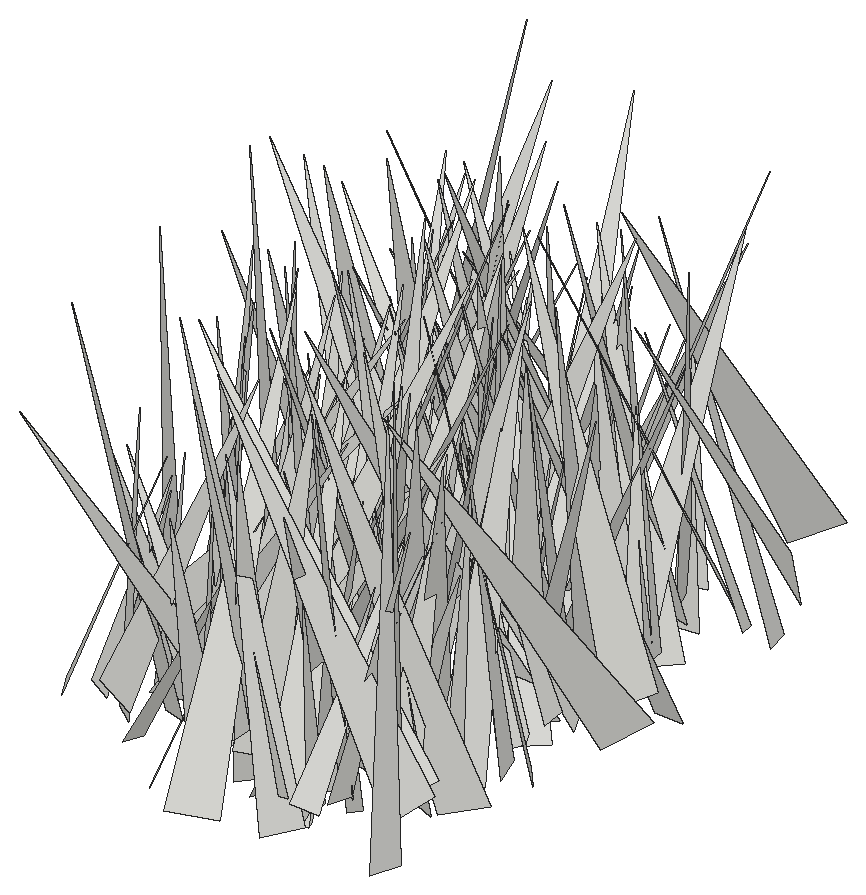
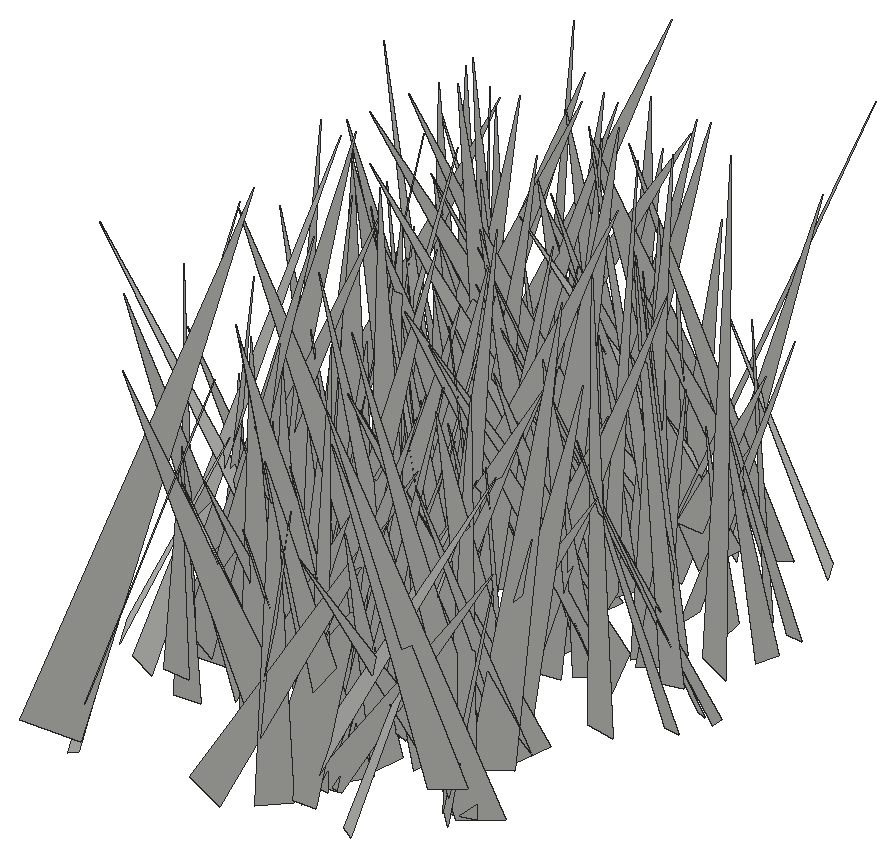
# SketchUp Ruby script. Lengths in inches.
U = 1.inch
M = Sketchup.active_model
def pt(a) = Geom::Point3d.new(a.map { |v| v * U })
def face(e, loops, mat)
  f = e.add_face(loops[0].map { |a| pt(a) })
  loops[1..].each { |l| e.add_face(l.map { |a| pt(a) }).erase! }
  f.material = f.back_material = mat if mat
  f
end
# faces: each face lists its corners as indices into pts; further lists are holes
def faces(e, pts, list, mat = nil) = list.each { |f| face(e, (f[0].is_a?(Array) ? f : [f]).map { |l| l.map { |i| pts[i] } }, mat) }
# xy, xz, yz: faces in a plane at the given z, y or x. An outline is a flat list of corners, or four numbers for a rectangle; further outlines are holes
def ring(l) = l.size == 4 ? [[l[0], l[1]], [l[2], l[1]], [l[2], l[3]], [l[0], l[3]]] : l.each_slice(2).to_a
def flat(e, list, mat, &to3) = list.each { |f| face(e, (f[0].is_a?(Array) ? f : [f]).map { |l| ring(l).map { |u, v| to3.(u, v) } }, mat) }
def xy(e, z, list, mat = nil) = flat(e, list, mat) { |x, y| [x, y, z] }
def xz(e, y, list, mat = nil) = flat(e, list, mat) { |x, z| [x, y, z] }
def yz(e, x, list, mat = nil) = flat(e, list, mat) { |y, z| [x, y, z] }
def lines(e, pts, list) = list.each { |a, b| e.add_line(pt(pts[a]), pt(pts[b])) }
# prism: a flat outline (further loops are holes) pulled along v
def prism(e, loops, v, mat = nil)
  f = face(e, loops, mat); d = Geom::Vector3d.new(v.map { |x| x * U })
  f.pushpull(f.normal.samedirection?(d) ? d.length : -d.length)
end
def box(e, o, s, mat = nil) = prism(e, [[o, [o[0] + s[0], o[1], o[2]], [o[0] + s[0], o[1] + s[1], o[2]], [o[0], o[1] + s[1], o[2]]]], [0, 0, s[2]], mat)
def at(x, y, z, deg = 0) = Geom::Transformation.translation(pt([x, y, z])) * Geom::Transformation.rotation(ORIGIN, Z_AXIS, deg.degrees)
def axes(o, x, y, z) = Geom::Transformation.new([*x, 0, *y, 0, *z, 0, *pt(o).to_a, 1])
def part(name) = M.definitions.add(name)
# library, detail: a bought-in or finely detailed component or shape, given as its bounding box
def library(name, o, s) = part(name).tap { |d| box(d.entities, o, s) }
def detail(e, o, s) = box(e.add_group.entities, o, s)
def put(e, d, t, mat = nil) = e.add_instance(d, t).tap { |i| i.material = mat if mat }
def group(e, t, mat = nil) = e.add_group.tap { |g| g.transformation = t; g.material = mat if mat }.entities
root = M.entities
c1 = part("fur_instance\#9")
p = [[0.8125,0,1.79],[0.67,-0.02,1.48],[0,-0.11,0],[0,0.11,0]]
faces(c1.entities,p,[[0,1,2,3]])
put(root,c1,axes([144.91,70.6,-28.22],[-4.86777,3.35697,1.6535],[3.6105,4.92638,0.62739],[0.98366,-1.46972,5.8797]))
put(root,c1,axes([144.56,70.66,-27.1],[0.81184,5.62301,2.88886],[5.96448,-1.64652,1.52868],[-2.09495,-2.50871,5.47179]))
put(root,c1,axes([140.2,74.88,-28.22],[-6.95908,-3.88864,0.42907],[-3.38575,6.42493,3.31533],[1.96017,-2.70799,7.24975]))
put(root,c1,axes([140.84,72,-27.1],[2.96444,-3.24193,0.90441],[-3.19075,-3.09049,-0.61962],[-1.07107,0.23387,4.34903]))
put(root,c1,axes([148.3125,72.37,-27.1],[-7.32197,2.2534,1.35544],[2.57225,6.97064,2.30649],[0.54639,-2.61889,7.30542]))
put(root,c1,axes([142.36,72.67,-28.22],[4.51111,-4.76568,1.07484],[-4.75985,-4.61702,-0.49408],[-1.1004,0.43419,6.54353]))
put(root,c1,axes([144.95,72.11,-28.22],[3.93197,-0.07434,1.3447],[0.21137,-4.06439,-0.84276],[-1.33006,-0.86567,3.84131]))
put(root,c1,axes([145.8125,72.4,-27.1],[3.71105,4.69804,3.51461],[5.68502,-3.90755,-0.77947],[-1.45074,-3.29476,5.93598]))
put(root,c1,axes([139.26,70.68,-27.1],[4.45979,0.0367,0.09292],[0.01604,-4.35825,0.95137],[-0.0986,0.95079,4.35729]))
put(root,c1,axes([141.31,71.35,-27.1],[2.46567,3.17158,1.58955],[3.37143,-2.69731,0.15219],[-1.10413,-1.15357,4.01439]))
put(root,c1,axes([143.47,68.16,-27.1],[-6.01479,5.28528,0.0687],[5.03484,5.76049,-2.36301],[1.60915,1.73181,7.65037]))
put(root,c1,axes([143.72,74.79,-27.1],[5.51839,-2.97407,0.09463],[-2.75984,-5.19025,-2.17974],[-1.11235,-1.87694,5.87762]))
put(root,c1,axes([143.98,71.49,-27.1],[0.77097,6.55392,2.92574],[6.60675,-1.79779,2.28627],[-2.8044,-2.43357,6.19042]))
put(root,c1,axes([148.7,70.69,-28.22],[-6.72767,0.28008,1.7782],[-0.11729,6.79671,-1.51427],[1.7963,1.49276,6.56102]))
put(root,c1,axes([146.28,71.55,-27.1],[4.52049,-0.19473,1.20973],[-0.39564,-4.60837,0.73662],[-1.15967,0.81315,4.46432]))
put(root,c1,axes([145.81,70.5,-27.1],[-1.08496,4.24211,0.2137],[4.12597,1.10497,-0.98676],[1.00871,0.04308,4.26602]))
put(root,c1,axes([145.03,71.22,-28.22],[3.71678,-0.58843,1.31141],[-0.99782,-3.67326,1.17982],[-1.0346,1.42876,3.57333]))
put(root,c1,axes([135.72,71.87,-27.1],[3.83341,2.26597,0.28943],[2.28132,-3.82668,-0.25597],[-0.11822,-0.36786,4.44568]))
put(root,c1,axes([139.32,72.52,-27.1],[-3.64938,-5.29226,1.74557],[-5.55344,3.28039,-1.66476],[-0.463,2.36729,6.20923]))
put(root,c1,axes([144.82,72.98,-27.1],[5.44749,2.02001,0.26599],[2.02291,-5.27178,-1.39377],[0.24298,-1.39796,5.64031]))
put(root,c1,axes([137.25,72.32,-27.1],[1.94999,6.06367,1.85826],[6.06829,-1.21894,-2.39034],[1.84311,-2.40204,5.90397]))
put(root,c1,axes([142.7,72.15,-27.1],[-2.8521,5.31504,2.52319],[5.50682,3.39878,-0.93481],[2.07151,-1.71732,5.95905]))
put(root,c1,axes([147.66,73.25,-27.1],[-6.42815,4.45601,0.04956],[4.21627,6.0534,2.59983],[-1.44275,-2.16333,7.37686]))
put(root,c1,axes([144.63,70.98,-28.22],[-3.90742,5.66938,0.63215],[5.60395,3.95813,-0.85923],[1.06639,-0.02677,6.83166]))
put(root,c1,axes([147.5625,72.71,-27.1],[-5.47988,-2.79163,2.54101],[-3.31815,5.69792,-0.89593],[1.79996,2.00489,6.08438]))
put(root,c1,axes([148.27,74.91,-28.22],[1.94153,-7.03493,2.68991],[-6.84514,-2.80689,-2.40016],[-3.14163,1.7682,6.89195]))
put(root,c1,axes([136.88,73.22,-28.22],[2.79154,3.79561,1.789],[3.98615,-3.06992,0.29332],[-1.31064,-1.25251,4.70248]))
put(root,c1,axes([138.55,73.31,-27.1],[4.87522,-3.55324,0.35007],[-3.38958,-4.41978,2.34354],[1.12198,2.08707,5.55888]))
put(root,c1,axes([140.44,73.48,-28.22],[-2.74524,3.88345,0.46197],[3.73915,2.44095,1.70042],[-1.14601,-1.33847,4.4414]))
put(root,c1,axes([140.1,70.5,-28.22],[6.17595,4.1917,0.11311],[3.92557,-5.85042,2.46738],[-1.47413,1.98185,7.04448]))
put(root,c1,axes([141.51,72.01,-27.1],[3.64416,1.65962,0.06909],[1.4569,-3.27351,1.789],[-0.79783,1.60274,3.58241]))
put(root,c1,axes([147.36,74.18,-28.22],[-2.59622,-3.87524,1.56211],[-4.17566,2.47102,-0.8099],[0.14666,1.75346,4.59368]))
put(root,c1,axes([138.39,74.91,-28.22],[-4.93591,-0.64757,0.62999],[-0.58328,4.95621,0.52453],[0.68994,-0.44273,4.95049]))
put(root,c1,axes([135.37,73.94,-28.22],[1.6531,3.56586,0.9383],[3.65871,-1.45863,-0.90264],[0.45784,-1.21883,3.82535]))
put(root,c1,axes([144.48,73.38,-28.22],[4.39475,-2.24157,1.41228],[-2.61052,-4.13054,1.56743],[-0.4521,2.06082,4.67778]))
put(root,c1,axes([143.18,74.8,-27.1],[4.24569,0.44069,0.96407],[0.53821,-4.32495,-0.39327],[-0.91322,-0.50013,4.25034]))
put(root,c1,axes([146.86,73.67,-27.1],[3.58302,-2.92408,2.58959],[-3.63927,-3.77537,0.77237],[-1.41842,2.30013,4.5598]))
put(root,c1,axes([144.4,75.02,-28.22],[-2.18314,-4.32344,1.23175],[-4.48368,1.99494,-0.94459],[-0.32548,1.51774,4.75036]))
put(root,c1,axes([139.69,75.49,-27.1],[1.75829,5.41715,3.42251],[6.36736,-1.87488,-0.30363],[-0.71818,-3.36006,5.68726]))
put(root,c1,axes([141.34,73.91,-27.1],[2.97178,5.39968,0.42783],[5.06638,-2.59832,-2.39825],[1.91609,-1.5044,5.67771]))
put(root,c1,axes([135.1875,75.38,-28.22],[3.83276,-0.80553,0.30542],[-0.78769,-3.84079,-0.24507],[-0.34886,-0.17786,3.90882]))
put(root,c1,axes([141.13,72.51,-27.1],[1.53253,6.73152,0.42824],[6.72346,-1.5597,0.45586],[-0.5402,-0.31526,6.8887]))
put(root,c1,axes([145.4,76.66,-28.22],[-2.92587,-7.18113,1.16279],[-7.26033,2.80394,-0.95233],[-0.45638,1.43204,7.69561]))
put(root,c1,axes([145.78,72.88,-28.22],[-6.55777,-1.69063,0.96933],[-1.94723,5.82112,-3.02077],[0.07829,3.17151,6.06115]))
put(root,c1,axes([145.0625,77.21,-28.22],[6.03142,-3.81553,0.06105],[-3.78285,-5.99326,-0.84318],[-0.50203,-0.68018,7.08699]))
put(root,c1,axes([143.54,74.2,-28.22],[3.01287,6.59159,3.14785],[6.68601,-3.85992,1.68335],[-2.94198,-2.02171,7.04931]))
put(root,c1,axes([143.01,72.125,-28.22],[8.13391,1.72844,0.70897],[1.41113,-7.75982,2.72846],[-1.22428,2.53935,7.85515]))
put(root,c1,axes([144.18,77.49,-28.22],[1.32188,-7.44707,0.58602],[-7.30684,-1.16527,1.67389],[1.55318,0.85612,7.37593]))
put(root,c1,axes([143.18,77.08,-27.1],[7.23074,-0.77372,0.74856],[-0.57311,-7.06946,-1.77111],[-0.91134,-1.69312,7.05304]))
put(root,c1,axes([137.75,77.37,-28.22],[5.72206,-2.67718,0.30846],[-2.55509,-5.6197,-1.37653],[-0.85672,-1.12072,6.16558]))
put(root,c1,axes([137.01,74.78,-28.22],[-3.53887,0.08812,1.47041],[-0.2173,3.75324,-0.74791],[1.45693,0.77383,3.46005]))
put(root,c1,axes([138.84,75.36,-28.22],[6.97385,3.06548,2.09729],[3.25235,-7.19468,-0.2986],[-1.79388,-1.12684,7.61201]))
put(root,c1,axes([139.07,74.93,-28.22],[3.68214,4.39884,2.0354],[4.4735,-4.06815,0.69917],[-1.86561,-1.07294,5.69378]))
put(root,c1,axes([145.66,77.23,-28.22],[-6.33507,2.2676,3.27677],[3.13305,6.63723,1.4641],[2.46237,-2.61105,6.56746]))
put(root,c1,axes([144.6875,76.66,-28.22],[2.13927,-3.81253,0.27989],[-3.71667,-1.99926,1.17453],[0.89447,0.81104,4.21098]))
put(root,c1,axes([136.02,76.74,-28.22],[3.79237,5.90894,3.79832],[6.9076,-3.92109,-0.79686],[-1.27587,-3.6653,6.97586]))
put(root,c1,axes([145.86,74.5,-28.22],[-3.10832,3.75001,0.92239],[3.63037,3.24121,-0.94342],[1.31674,-0.08395,4.77852]))
put(root,c1,axes([141.09,74.19,-27.1],[-0.22471,7.89617,1.63504],[7.5306,0.79034,-2.78188],[2.88322,-1.44886,7.39332]))
put(root,c1,axes([143.5625,74.51,-28.22],[4.95008,1.27612,1.12304],[0.89586,-4.89693,1.61571],[-1.4447,1.33589,4.84988]))
put(root,c1,axes([147.38,75.45,-28.22],[1.56469,4.5597,1.40699],[4.65343,-1.78584,0.61247],[-1.05645,-1.11294,4.78163]))
put(root,c1,axes([143.38,76.67,-27.1],[1.79677,-5.19077,1.98742],[-5.55817,-1.66844,0.66734],[0.02536,2.09632,5.45226]))
put(root,c1,axes([144.99,74.91,-27.1],[-0.16365,8.04006,1.71484],[8.20749,0.06185,0.49328],[-0.46944,-1.72152,8.02659]))
put(root,c1,axes([137.49,77.74,-28.22],[3.23004,-2.47849,1.2151],[-2.38486,-3.44753,-0.69249],[-1.3899,0.15559,4.01205]))
put(root,c1,axes([143.25,76.32,-27.1],[-2.90723,2.3787,0.42473],[2.40963,2.90345,0.23285],[0.1797,-0.4498,3.74913]))
put(root,c1,axes([139.47,76.58,-27.1],[-3.40994,2.09099,1.78678],[2.1335,3.80705,-0.3836],[1.73581,-0.57158,3.98156]))
put(root,c1,axes([146.58,80.24,-28.22],[1.87232,-8.06563,0.81969],[-7.60481,-2.03883,-2.69107],[-2.80947,0.14362,7.83059]))
put(root,c1,axes([147.76,77.57,-28.22],[4.40996,1.53054,2.75088],[1.88618,-5.07543,-0.19988],[-2.52036,-1.1203,4.66373]))
put(root,c1,axes([143.81,78.94,-27.1],[7.53646,1.85279,1.2332],[2.16443,-7.11553,-2.53698],[-0.51849,-2.77277,7.33449]))
put(root,c1,axes([137.88,76.2,-28.22],[2.58836,6.22661,1.98748],[6.38761,-2.86286,0.6503],[-1.38536,-1.56644,6.71174]))
put(root,c1,axes([149.2,81.38,-28.22],[4.76692,-6.38187,0.99404],[-5.33821,-4.5884,-3.85875],[-3.63592,-1.6304,6.96863]))
put(root,c1,axes([148.56,77.71,-28.22],[-5.72763,-4.55632,1.57593],[-4.80185,5.61014,-1.23206],[0.43111,1.95337,7.21442]))
put(root,c1,axes([143.7,78.13,-27.1],[-6.59669,1.20746,2.1658],[1.44471,6.87425,0.5679],[2.0153,-0.97558,6.6822]))
put(root,c1,axes([142.8,75.98,-27.1],[-0.26987,6.47949,0.83868],[6.52839,0.23411,0.29205],[-0.25936,-0.84936,6.47853]))
put(root,c1,axes([139.97,80.08,-28.22],[1.76512,-7.95634,1.31885],[-8.03843,-1.84494,-0.37166],[-0.65291,1.20466,8.14131]))
put(root,c1,axes([147.1875,75.96,-28.22],[5.43527,-3.00495,4.38513],[-4.48513,-5.95873,1.47596],[-2.85354,3.64214,6.0327]))
put(root,c1,axes([139.26,77.5625,-27.1],[-7.32615,-2.19993,2.60741],[-2.57876,7.61493,-0.82074],[2.23345,1.57604,7.60517]))
put(root,c1,axes([143.94,77.67,-28.22],[0.54119,7.40359,2.44886],[7.61955,0.0202,-1.74498],[1.65906,-2.50787,7.21533]))
put(root,c1,axes([135.09,79.8125,-27.1],[-1.49518,-5.85947,1.8909],[-5.5495,2.12534,2.19783],[2.66683,1.13753,5.63369]))
put(root,c1,axes([141.99,74.95,-27.1],[7.42778,3.7642,0.92799],[3.25227,-7.14156,2.93652],[-2.11023,2.24305,7.79217]))
put(root,c1,axes([134,79.12,-28.22],[4.7067,5.43888,0.18038],[4.50837,-3.76361,-4.15655],[3.04771,-2.83211,5.87006]))
put(root,c1,axes([148.11,79.28,-27.1],[-3.79704,-0.30553,0.54536],[-0.26679,3.82814,0.28712],[0.56533,-0.2455,3.79848]))
put(root,c1,axes([147.06,78.76,-28.22],[-4.286,2.05614,0.85108],[2.13965,4.31523,0.34994],[0.6115,-0.68765,4.74078]))
put(root,c1,axes([141.41,77.72,-27.1],[-2.96108,3.10315,0.36366],[3.04624,2.97875,-0.6142],[0.69442,0.16515,4.24503]))
put(root,c1,axes([134.65,79.04,-28.22],[5.32286,5.30667,0.20638],[4.93366,-4.8331,-2.97258],[1.96528,-2.23975,6.90343]))
put(root,c1,axes([140.23,77.92,-28.22],[-1.52341,4.48001,0.30788],[4.47725,1.54034,-0.26007],[0.34571,-0.20714,4.72479]))
put(root,c1,axes([147.53,81.13,-28.22],[-3.34335,-1.51871,0.13226],[-1.40215,3.18862,1.16988],[0.59829,-1.01398,3.48078]))
put(root,c1,axes([145.8,80.96,-28.22],[1.85268,-6.56464,1.39244],[-6.70428,-1.74747,0.68181],[0.2934,1.52239,6.78691]))
put(root,c1,axes([144.1,79.8125,-27.1],[5.56182,2.46032,2.03104],[2.73268,-5.78042,-0.48104],[-1.64644,-1.28288,6.06264]))
put(root,c1,axes([139.77,77.98,-28.22],[-5.38629,2.97439,0.98855],[2.72826,5.41671,-1.43257],[1.54299,0.80541,5.98388]))
put(root,c1,axes([137.07,80.18,-28.22],[3.3764,2.66955,0.1135],[2.47122,-3.05035,-1.76859],[1.01611,-1.452,3.92412]))
put(root,c1,axes([139.67,80.86,-27.1],[-1.62801,-6.13851,1.48062],[-6.15059,1.19536,-1.80699],[-1.42958,1.84764,6.08822]))
put(root,c1,axes([146.36,80.59,-27.1],[5.46664,-0.56538,0.68203],[-0.51758,-5.49848,-0.40957],[-0.71898,-0.34055,5.48051]))
put(root,c1,axes([142.17,78.28,-27.1],[-2.25135,6.36064,1.32657],[6.19225,2.52565,-1.60099],[1.96812,-0.67041,6.55463]))
put(root,c1,axes([138.54,79.36,-28.22],[-1.83169,3.1238,0.57494],[3.14275,1.87858,-0.19441],[0.4602,-0.39568,3.61599]))
put(root,c1,axes([142.43,78.56,-28.22],[1.48106,4.37962,0.44895],[4.22706,-1.54701,1.14671],[-1.23071,-0.04293,4.4788]))
put(root,c1,axes([138.99,78.66,-27.1],[-4.17558,2.72173,1.55923],[2.19552,4.39009,-1.78362],[2.24025,0.77057,4.65424]))
put(root,c1,axes([146.53,81.85,-27.1],[-2.50316,-5.2047,1.47138],[-5.2002,2.76171,0.92225],[1.48721,0.89649,5.70124]))
put(root,c1,axes([136.28,81.58,-28.22],[-2.31612,-6.1908,2.36322],[-6.27799,2.85121,1.3163],[2.12077,1.67923,6.47748]))
put(root,c1,axes([143.03,81.9,-27.1],[1.51569,-5.39227,1.25729],[-5.41404,-1.71643,-0.83467],[-1.15995,0.96539,5.5387]))
put(root,c1,axes([134.71,80.3,-28.22],[2.35379,3.88662,0.95748],[3.9563,-2.09005,-1.24191],[0.60851,-1.44527,4.3708]))
put(root,c1,axes([145.65,82.99,-28.22],[-6.24986,-4.52728,1.84324],[-4.17742,6.50052,1.80193],[2.5383,-0.44892,7.504]))
put(root,c1,axes([147.33,79.15,-28.22],[-3.60755,4.52257,0.00535],[4.517,3.60276,0.29145],[-0.22451,-0.18592,5.77782]))
put(root,c1,axes([142.91,81.48,-27.1],[-7.09229,4.18803,1.11711],[4.32642,6.70959,2.31334],[-0.26383,-2.55536,7.90497]))
put(root,c1,axes([140.57,76.53,-28.22],[-6.04626,5.73242,0.3376],[5.11125,5.59588,-3.47751],[2.61721,2.31459,7.57131]))
put(root,c1,axes([146.88,82.53,-27.1],[6.67439,0.3641,2.55328],[0.99441,-6.8993,-1.61558],[-2.3797,-1.86182,6.48614]))
put(root,c1,axes([139.86,83.11,-27.1],[-1.86711,-6.21996,0.83765],[-6.21183,1.95621,0.67975],[0.89595,0.60083,6.45848]))
put(root,c1,axes([145.15,81.35,-27.1],[3.94564,1.0984,0.79467],[1.2,-3.96752,-0.47419],[-0.63087,-0.67703,4.06813]))
put(root,c1,axes([149.29,81.51,-27.1],[-7.00283,2.97011,1.6591],[3.21934,7.01289,1.03394],[1.10002,-1.61605,7.53606]))
put(root,c1,axes([141.0625,81.28,-28.22],[-2.95637,3.32548,0.26078],[3.10336,2.61427,1.84435],[-1.22309,-1.40488,4.04936]))
put(root,c1,axes([139.37,83.22,-27.1],[1.40326,-4.201,0.43994],[-3.89786,-1.46649,-1.57071],[-1.62745,-0.10993,4.1413]))
put(root,c1,axes([149.48,82.98,-28.22],[-2.28095,-6.51713,0.89519],[-6.46928,2.05047,-1.55597],[-1.19279,1.34151,6.72716]))
put(root,c1,axes([146.16,79.88,-28.22],[1.52611,3.71718,0.33458],[3.41655,-1.5369,1.49113],[-1.50217,0.28087,3.73135]))
put(root,c1,axes([137.89,78.65,-28.22],[6.68377,2.4417,1.0502],[1.89436,-6.36953,2.75283],[-1.86446,2.28139,6.56175]))
put(root,c1,axes([143,83.0625,-28.22],[-4.99483,-3.69291,1.05885],[-3.66459,5.10128,0.50484],[1.15306,0.21561,6.19121]))
put(root,c1,axes([144.1875,81.26,-27.1],[3.38997,4.6985,2.258],[4.82742,-3.84601,0.75539],[-1.96736,-1.34115,5.74432]))
put(root,c1,axes([139.67,83.43,-28.22],[3.51302,-4.23345,1.0034],[-4.35037,-3.40123,0.88101],[0.05668,1.33409,5.43021]))
put(root,c1,axes([140.08,83.51,-27.1],[6.22111,3.48137,1.76986],[3.77865,-6.20685,-1.07301],[-0.98698,-1.81924,7.04775]))
put(root,c1,axes([141.17,85.9,-28.22],[4.72004,-5.82808,0.22381],[-5.80637,-4.72269,-0.52693],[-0.55017,-0.15829,7.48115]))
put(root,c1,axes([138.85,83.3,-27.1],[4.00395,3.96639,1.91354],[4.25291,-4.1539,-0.28869],[-1.14309,-1.56151,5.62855]))
put(root,c1,axes([141.91,82.83,-28.22],[-0.29437,7.39176,2.68978],[7.28817,1.26884,-2.68928],[2.95898,-2.3899,6.89148]))
put(root,c1,axes([143.33,82.87,-28.22],[-4.54084,5.90887,0.08971],[5.53212,4.21055,2.68494],[-2.07809,-1.7025,6.95162]))
put(root,c1,axes([142.61,84.73,-27.1],[0.82361,-5.861,1.93807],[-5.93962,-1.28507,-1.3621],[-1.68178,1.66825,5.75972]))
put(root,c1,axes([138.26,83.41,-28.22],[-5.76808,3.66085,1.08427],[3.77252,5.76709,0.59739],[0.58783,-1.08949,6.80556]))
put(root,c1,axes([147.86,83.56,-28.22],[-2.40866,3.6867,1.3913],[3.88066,2.50239,0.08743],[0.68406,-1.21467,4.40293]))
put(root,c1,axes([145.04,82.98,-28.22],[5.62442,0.34622,0.61815],[0.22701,-5.5658,1.05184],[-0.67115,1.01884,5.53603]))
put(root,c1,axes([137.65,84.18,-27.1],[-2.04031,-2.94511,1.87891],[-3.25881,2.38849,0.20512],[1.25863,1.41005,3.57693]))
put(root,c1,axes([138.14,86.42,-27.1],[6.98441,-2.34407,2.00985],[-1.86712,-7.16517,-1.86827],[-2.45928,-1.21733,7.12645]))
put(root,c1,axes([141.48,86.75,-27.1],[3.03189,-3.59681,0.02756],[-3.43565,-2.90654,-1.37057],[-1.06494,-0.8632,4.50011]))
put(root,c1,axes([143.98,86,-27.1],[3.85722,-2.97975,0.1804],[-2.96484,-3.85827,-0.33622],[-0.3481,-0.15623,4.86251]))
put(root,c1,axes([142.22,84.82,-27.1],[-4.50006,-1.01814,0.39176],[-1.03948,4.50642,-0.22865],[0.331,0.31016,4.60813]))
put(root,c1,axes([147.51,88.26,-27.1],[-4.65731,-6.85842,0.0184],[-6.74044,4.58127,1.51895],[1.26677,-0.83835,8.14992]))
put(root,c1,axes([136.05,86.8,-27.1],[5.91516,-3.3432,1.65321],[-2.9566,-6.09276,-1.74243],[-2.27346,-0.77492,6.56735]))
put(root,c1,axes([143.23,84.64,-27.1],[0.75971,3.71481,1.88794],[3.89435,-1.31575,1.02184],[-1.48263,-1.55251,3.65142]))
put(root,c1,axes([138.7,83.67,-28.22],[-4.67353,1.04438,0.03845],[1.02272,4.60667,-0.8165],[0.21505,0.78861,4.71868]))
put(root,c1,axes([146.2,84.99,-27.1],[-4.24357,2.27798,1.78244],[2.54082,4.44811,0.36434],[1.38223,-1.18292,4.80254]))
put(root,c1,axes([140.07,86.27,-27.1],[6.97183,-3.45055,1.53762],[-3.37643,-7.13932,-0.71191],[-1.69419,0.0288,7.74635]))
put(root,c1,axes([148.16,83.91,-27.1],[-6.10428,-1.79449,1.71008],[-2.20054,6.01533,-1.54278],[1.14113,2.0006,6.1727]))
put(root,c1,axes([139.66,86.74,-27.1],[-1.20375,-5.21342,0.24756],[-5.17288,1.15789,-0.76855],[-0.69453,0.4118,5.2951]))
put(root,c1,axes([137.97,83.47,-27.1],[5.78446,0.51407,0.77192],[0.25637,-5.57234,1.78981],[-0.89129,1.73346,5.52457]))
put(root,c1,axes([139.04,82.79,-28.22],[-3.85678,5.81728,0.33644],[5.7739,3.8696,-0.71896],[0.78484,0.11882,6.94252]))
put(root,c1,axes([147.09,86.22,-27.1],[-2.90211,-6.23156,1.67253],[-6.44447,2.71044,-1.08359],[-0.31368,1.96803,6.78825]))
put(root,c1,axes([142.2,85.97,-28.22],[-3.6362,-3.51378,0.23491],[-3.4583,3.49912,-1.19165],[-0.6648,1.01649,4.91412]))
put(root,c1,axes([135.7,85.43,-27.1],[4.06898,-3.86093,0.67624],[-3.71406,-3.48612,2.44405],[1.25293,2.20473,5.04877]))
put(root,c1,axes([143.81,84.67,-27.1],[3.84083,1.33111,0.88578],[1.09907,-3.87194,1.0529],[-1.16125,0.73803,3.92622]))
put(root,c1,axes([145.41,83.36,-27.1],[6.47525,4.61232,0.40047],[4.47579,-6.41261,1.48613],[-1.18373,0.98374,7.80985]))
put(root,c1,axes([147.35,85.29,-28.22],[-2.86561,6.0597,1.12131],[6.09085,2.59686,1.53195],[-0.93747,-1.65086,6.5257]))
put(root,c1,axes([136.34,87.87,-28.22],[-0.27546,-6.0552,1.07535],[-6.00995,0.49341,1.23885],[1.30474,0.99438,5.93351]))
put(root,c1,axes([146.55,87.375,-27.1],[5.52429,1.58059,2.16664],[1.98524,-5.74559,-0.8703],[-1.80317,-1.48335,5.67966]))
put(root,c1,axes([137.67,87.54,-27.1],[7.30646,0.41261,0.41525],[0.46932,-7.23653,-1.06747],[-0.34987,-1.09065,7.23983]))
put(root,c1,axes([143.98,87.33,-27.1],[-0.35504,-4.51922,1.36303],[-4.31721,-0.2418,-1.92625],[-1.90863,1.3876,4.10353]))
put(root,c1,axes([146.66,84.76,-27.1],[-1.23708,6.4323,0.84499],[6.38548,1.35924,-0.99849],[1.14637,-0.62994,6.47363]))
put(root,c1,axes([140.75,90.08,-28.22],[0.62863,-8.27068,0.12443],[-8.26435,-0.63324,-0.33804],[-0.34653,0.09834,8.28764]))
put(root,c1,axes([141.62,88.53,-28.22],[2.79879,-2.29313,0.37979],[-2.08936,-2.74248,-1.16161],[-1.01846,-0.6755,3.42672]))
put(root,c1,axes([145.6,86.17,-28.22],[3.61402,1.40651,0.81578],[1.29809,-3.69316,0.61679],[-0.97915,0.29527,3.8287]))
put(root,c1,axes([147.17,91.81,-28.22],[-5.2335,-6.40482,0.23356],[-5.52847,4.66397,4.0186],[3.24225,-2.38569,7.22925]))
put(root,c1,axes([140.25,87.83,-28.22],[-6.31827,-0.38458,1.65434],[-0.20418,6.49842,0.73085],[1.68614,-0.65417,6.28763]))
put(root,c1,axes([141.63,87.22,-27.1],[5.98361,0.11352,0.76596],[0.13466,-6.02993,-0.15823],[-0.76252,-0.17402,5.9826]))
put(root,c1,axes([141.55,85.85,-28.22],[4.20978,2.5999,1.29958],[2.36123,-4.39284,1.13935],[-1.69498,0.33775,4.81493]))
put(root,c1,axes([136.29,85.29,-27.1],[0.97806,5.36378,0.25201],[5.36787,-0.98334,0.09641],[-0.14015,-0.23057,5.45137]))
put(root,c1,axes([143.35,88.09,-27.1],[4.53528,-3.04969,1.17101],[-3.07507,-4.66168,-0.23091],[-1.10265,0.45689,5.46041]))
put(root,c1,axes([140.29,88.8,-28.22],[-1.9531,-3.93926,0.49775],[-3.87343,2.01224,0.72636],[0.87298,0.11511,4.33645]))
put(root,c1,axes([149.2,86.99,-27.1],[-4.27231,-1.94809,0.06255],[-1.87913,4.07681,-1.37844],[-0.51754,1.27912,4.48861]))
put(root,c1,axes([143.74,85.65,-27.1],[3.9731,1.20771,1.01378],[0.70264,-3.81635,1.79266],[-1.41159,1.49959,3.74573]))
put(root,c1,axes([146.57,87.4,-28.22],[-0.32853,3.96848,1.56907],[4.26678,0.33258,0.05223],[0.07349,-1.56822,3.98171]))
put(root,c1,axes([140.61,89.0625,-28.22],[-1.97091,-5.99186,1.73382],[-5.97714,2.33419,1.27215],[1.7839,1.20092,6.17807]))
put(root,c1,axes([136.53,88.26,-28.22],[-2.53419,-2.69204,0.92744],[-2.77792,2.61003,-0.01451],[0.6248,0.68554,3.69715]))
put(root,c1,axes([141.97,86.8125,-27.1],[-2.66965,3.73747,0.14274],[3.69986,2.61324,0.77338],[-0.54785,-0.56423,4.52743]))
put(root,c1,axes([143.28,84.67,-28.22],[-2.88963,7.72101,0.14725],[7.7077,2.8933,-0.45358],[0.4764,0.02131,8.23153]))
put(root,c1,axes([141.83,87.72,-27.1],[-5.56985,2.38046,0.65327],[2.45077,5.52546,0.76123],[0.29505,-0.95874,6.00918]))
put(root,c1,axes([139.78,86.84,-28.22],[3.76541,-0.98312,2.37268],[-1.72485,-4.08783,1.04352],[-1.9029,1.75998,3.74912]))
put(root,c1,axes([143.125,86.76,-28.22],[3.44436,3.22324,0.28553],[3.18394,-3.45028,0.54084],[-0.57733,0.20181,4.68619]))
put(root,c1,axes([136.98,86.49,-27.1],[7.21368,2.51232,2.17903],[2.05011,-7.45745,1.81123],[-2.61859,1.08246,7.42081]))
put(root,c1,axes([138.21,90.6,-28.22],[-3.05725,-3.63504,0.09512],[-3.51202,2.98398,1.15363],[0.94245,-0.67208,4.60753]))
put(root,c1,axes([140.33,88.97,-28.22],[-4.24155,2.82864,0.08548],[2.61337,3.85608,2.07369],[-1.08573,-1.76881,4.65744]))
put(root,c1,axes([146.46,88.02,-27.1],[-0.50007,3.75556,1.02909],[3.87876,0.38868,0.46638],[-0.34425,-1.07612,3.75989]))
put(root,c1,axes([147.2,92.79,-27.1],[4.97759,-6.71856,0.2944],[-6.18791,-4.7191,-3.07278],[-2.63353,-1.61035,7.77647]))
put(root,c1,axes([137.27,86.6875,-28.22],[4.79921,1.03907,0.41248],[0.79797,-4.45725,1.94381],[-0.78297,1.82633,4.50929]))
put(root,c1,axes([142.9,86.96,-27.1],[1.96135,3.70682,0.36248],[3.45553,-1.96392,1.38604],[-1.38968,0.34826,3.95807]))
put(root,c1,axes([139.96,88.15,-28.22],[-2.58112,4.19595,2.18678],[4.13957,3.20902,-1.27135],[2.29171,-1.07069,4.75939]))
put(root,c1,axes([140.96,89.26,-28.22],[-5.24888,-4.54366,0.15791],[-4.36596,4.97023,-2.11085],[-1.26815,1.69482,6.61361]))
put(root,c1,axes([149.1,88.54,-28.22],[-6.20853,-2.44848,0.56631],[-2.51301,6.03462,-1.45936],[-0.02325,1.56521,6.51238]))
put(root,c1,axes([140.87,90.6,-28.22],[4.92449,-2.5321,0.51516],[-2.43841,-4.92066,-0.87679],[-0.85503,-0.55051,5.46748]))
put(root,c1,axes([142.84,91.25,-28.22],[-0.84326,-5.89202,0.02664],[-5.53518,0.78295,-2.04363],[-2.01949,0.3143,5.59022]))
put(root,c1,axes([142.31,89.55,-27.1],[-3.28529,-1.60429,1.12724],[-1.66632,3.44368,0.04462],[1.03333,0.45264,3.6558]))
put(root,c1,axes([142.35,88.64,-27.1],[5.41003,-2.25588,0.78895],[-2.38957,-5.13634,1.69936],[-0.03699,1.87321,5.60977]))
put(root,c1,axes([135.73,87.66,-28.22],[-1.22058,7.14872,1.6543],[7.02907,1.62036,-1.81584],[2.10547,-1.26529,7.02116]))
put(root,c1,axes([136.34,88.39,-27.1],[-0.72846,5.64896,1.65026],[5.62241,1.15927,-1.48642],[1.73859,-1.38206,5.49837]))
